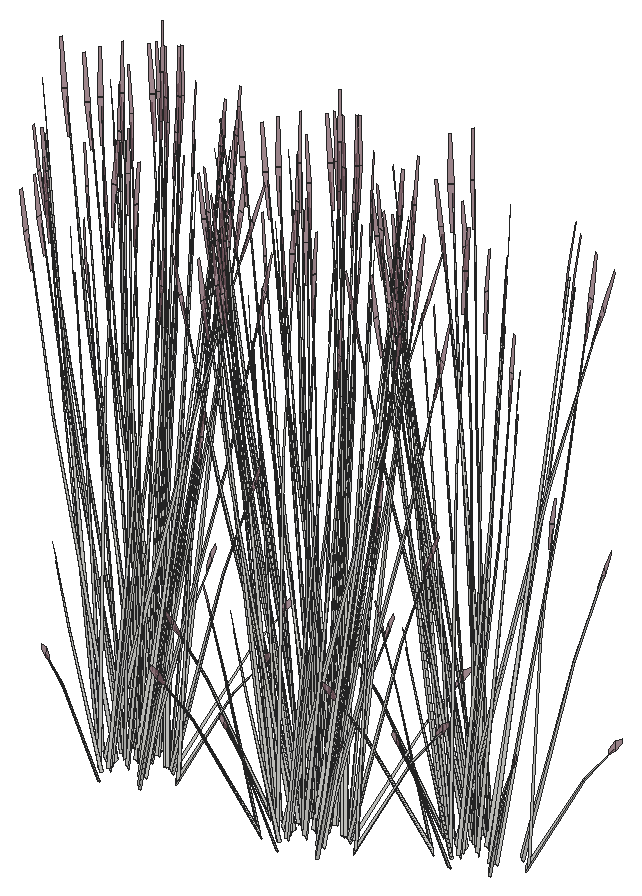
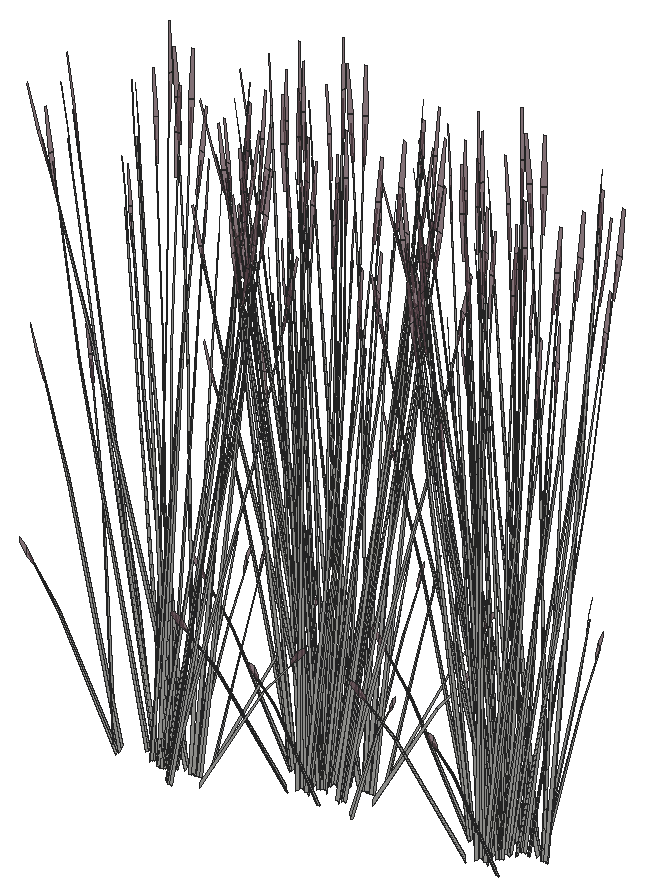
# SketchUp Ruby script. Lengths in inches.
U = 1.inch
M = Sketchup.active_model
def pt(a) = Geom::Point3d.new(a.map { |v| v * U })
def face(e, loops, mat)
  f = e.add_face(loops[0].map { |a| pt(a) })
  loops[1..].each { |l| e.add_face(l.map { |a| pt(a) }).erase! }
  f.material = f.back_material = mat if mat
  f
end
# faces: each face lists its corners as indices into pts; further lists are holes
def faces(e, pts, list, mat = nil) = list.each { |f| face(e, (f[0].is_a?(Array) ? f : [f]).map { |l| l.map { |i| pts[i] } }, mat) }
# xy, xz, yz: faces in a plane at the given z, y or x. An outline is a flat list of corners, or four numbers for a rectangle; further outlines are holes
def ring(l) = l.size == 4 ? [[l[0], l[1]], [l[2], l[1]], [l[2], l[3]], [l[0], l[3]]] : l.each_slice(2).to_a
def flat(e, list, mat, &to3) = list.each { |f| face(e, (f[0].is_a?(Array) ? f : [f]).map { |l| ring(l).map { |u, v| to3.(u, v) } }, mat) }
def xy(e, z, list, mat = nil) = flat(e, list, mat) { |x, y| [x, y, z] }
def xz(e, y, list, mat = nil) = flat(e, list, mat) { |x, z| [x, y, z] }
def yz(e, x, list, mat = nil) = flat(e, list, mat) { |y, z| [x, y, z] }
def lines(e, pts, list) = list.each { |a, b| e.add_line(pt(pts[a]), pt(pts[b])) }
# prism: a flat outline (further loops are holes) pulled along v
def prism(e, loops, v, mat = nil)
  f = face(e, loops, mat); d = Geom::Vector3d.new(v.map { |x| x * U })
  f.pushpull(f.normal.samedirection?(d) ? d.length : -d.length)
end
def box(e, o, s, mat = nil) = prism(e, [[o, [o[0] + s[0], o[1], o[2]], [o[0] + s[0], o[1] + s[1], o[2]], [o[0], o[1] + s[1], o[2]]]], [0, 0, s[2]], mat)
def at(x, y, z, deg = 0) = Geom::Transformation.translation(pt([x, y, z])) * Geom::Transformation.rotation(ORIGIN, Z_AXIS, deg.degrees)
def axes(o, x, y, z) = Geom::Transformation.new([*x, 0, *y, 0, *z, 0, *pt(o).to_a, 1])
def part(name) = M.definitions.add(name)
# library, detail: a bought-in or finely detailed component or shape, given as its bounding box
def library(name, o, s) = part(name).tap { |d| box(d.entities, o, s) }
def detail(e, o, s) = box(e.add_group.entities, o, s)
def put(e, d, t, mat = nil) = e.add_instance(d, t).tap { |i| i.material = mat if mat }
def group(e, t, mat = nil) = e.add_group.tap { |g| g.transformation = t; g.material = mat if mat }.entities
root = M.entities
M.materials.add("LightPink_Translucent").color = [144, 107, 117]
M.materials["LightPink_Translucent"].alpha = 0.75
c1 = part("blade")
p = [[2.15,0.21,22],[0,0.17,0],[0.09,0.45,0],[2.18,0.31,22],[2.29,0.31,22],[0.38,0.45,0],
  [2.48,0.24,33],[2.49,0.24,33],[2.48,0.22,33]]
faces(c1.entities,p,[[0,1,2,3],[4,5,2,3],[6,3,4,7],[8,0,3,6]])
c2 = part("seeds")
p = [[0.3,-0.1,1.38],[-0.01,-0.03,1.59],[-0.01,-0.03,0.03],[0.14,-0.07,-0.07],[0.29,-0.03,3],[0.15,0.01,3.11]]
faces(c2.entities,p,[[0,1,2,3],[1,0,4,5]],"LightPink_Translucent")
c3 = part("blade with seeds")
put(c3.entities,c1,at(0,0,0))
put(c3.entities,c2,axes([2.4,0.25,30.99],[1.5799,-0.05474,1.17369],[-0.12525,1.92788,0.29478],[-0.07173,-0.02425,1.56792]))
put(root,c3,axes([362.03,53.35,257.33],[-0.70674,0.51372,0.30756],[-0.70717,-0.50832,-0.36492],[-0.02468,-0.14589,1.64885]))
put(root,c3,axes([365.23,54.6,257.46],[-0.74193,-0.49181,-0.25192],[0.6243,-0.55226,0.5513],[-0.19979,0.05753,1.68216]))
put(root,c3,axes([363.88,54.13,257.21],[-0.45644,-0.51287,-0.44739],[0.69137,-0.36116,0.21531],[-0.14771,-0.06346,1.43643]))
put(root,c3,axes([364.85,54.5,257.21],[-0.82508,0.03772,-0.44739],[-0.07462,-0.62614,0.21531],[-0.14771,0.06346,1.43643]))
put(root,c3,axes([363.94,54.42,257.4375],[0.20138,-0.72405,-0.23429],[0.95485,0.12621,0.51271],[-0.16685,-0.09999,1.5644]))
put(root,c3,axes([365.72,56.11,257.02],[-0.7111,0.30552,-0.49651],[-0.42504,-0.54784,0],[-0.16196,0.06958,1.57504]))
put(root,c3,axes([361.51,53.07,257.02],[0,-0.61104,-0.49651],[0.85008,0,0],[0,-0.13917,1.57504]))
put(root,c3,axes([365.76,55.95,257.19],[-0.46912,-0.61443,-0.05142],[0.79476,-0.34146,0.51607],[-0.19584,0.0585,1.6363]))
put(root,c3,axes([365.55,55.87,257.03],[-0.70886,-0.15119,-0.30978],[0.17848,-0.53243,0.30978],[-0.1429,0.0614,1.38974]))
put(root,c3,axes([363.73,53.77,257.67],[-0.85568,-0.29155,-0.29095],[0.41201,-0.61537,-0.50002],[-0.02689,-0.15109,1.59708]))
put(root,c3,axes([365.43,54.33,257.67],[0.08854,0.69723,-0.29095],[-0.92215,0.04216,-0.50002],[-0.16238,0.09287,1.59708]))
put(root,c3,axes([363.35,53.15,257.1],[-0.31203,-0.62659,-0.69835],[0.89884,-0.22566,-0.18329],[-0.03449,-0.21218,1.54149]))
put(root,c3,axes([361.87,53.08,257.03],[0.53038,-0.38124,-0.30978],[0.53038,0.38124,0.30978],[0,-0.1228,1.38974]))
put(root,c3,axes([364.27,50.62,257.13],[-0.52505,0.35054,-0.03893],[-0.48109,-0.38392,-0.17649],[-0.03387,-0.10878,0.58215]))
put(root,c3,axes([364.59,55.33,257.2],[-0.76598,-0.27433,0],[0.36864,-0.57001,0],[0,0,1.62707]))
put(root,c3,axes([366.36,56.02,257.375],[0.47504,0.61229,0],[-0.79476,0.34146,-0.51607],[-0.18101,0.07777,1.63711]))
put(root,c3,axes([365.4,54.01,257.3],[-0.70674,-0.52593,-0.06131],[0.70717,-0.52625,0],[-0.02468,-0.01837,1.75571]))
put(root,c3,axes([365.78,55.63,257.33],[0.95122,0.19861,0.30756],[-0.23797,0.7099,-0.36492],[-0.15744,0.08885,1.64885]))
put(root,c3,axes([364.4,50.1875,256.49],[-0.12744,0.02202,1.76342],[-0.70477,-0.24781,-0.26939],[0.01183,-0.2067,0.30037]))
put(root,c3,axes([363.82,53.32,257.21],[0.36864,-0.55059,-0.44739],[0.76598,0.26498,0.21531],[0,-0.12692,1.43643]))
put(root,c3,axes([364.76,55.09,257.2],[-0.24791,-0.5268,0],[0.70791,-0.18448,0],[0,0,1.54371]))
put(root,c3,axes([363.86,56.2,256.49],[0.12297,-0.03325,1.76342],[0.73967,0.18301,-0.26939],[0.02163,0.20626,0.30037]))
put(root,c3,axes([365.76,54.05,257.21],[-0.36864,0.55059,-0.44739],[-0.76598,-0.26498,0.21531],[0,0.12692,1.43643]))
put(root,c3,axes([365.16,53.46,257.21],[0,-0.70701,0],[0.95008,0,0],[0,0,1.79456]))
put(root,c3,axes([365.64,53.74,257.29],[0,0.70667,-0.05637],[-0.95008,0,0],[0,0.02221,1.79368]))
put(root,c3,axes([365.18,55.11,257.29],[0.33034,0.70197,-0.06012],[-0.94388,0.24598,0],[0.01154,0.02451,1.72173]))
put(root,c3,axes([363.22,51.35,257.375],[-0.47504,-0.61229,0],[0.79476,-0.34146,-0.51607],[0.18101,-0.07777,1.63711]))
put(root,c3,axes([367.91,54.19,257.2],[-0.94962,-0.00489,-0.04976],[0,-0.68292,0.49943],[-0.02984,0.15546,1.58352]))
put(root,c3,axes([365.79,53.89,257.21],[0.53038,0.39469,0],[-0.53038,0.39469,0],[0,0,1.69266]))
put(root,c3,axes([365.46,55.34,257.2],[0.76598,0.27433,0],[-0.36864,0.57001,0],[0,0,1.74954]))
put(root,c3,axes([367.71,54.29,257.03],[-0.53038,0.38124,-0.30978],[-0.53038,-0.38124,0.30978],[0,0.1228,1.38974]))
put(root,c3,axes([366.2,54.22,257.09],[0.2786,0.55945,-0.69212],[-0.80253,0.20149,-0.18165],[0.03079,0.18945,1.52773]))
put(root,c3,axes([365.8,53.62,257.21],[0.85008,0,0],[0,0.63259,0],[0,0,1.78407]))
put(root,c3,axes([364.16,53.04,257.67],[-0.08854,-0.69723,-0.29095],[0.92215,-0.04216,-0.50002],[0.16238,-0.09287,1.59708]))
put(root,c3,axes([365.86,53.6,257.67],[0.85568,0.29155,-0.29095],[-0.41201,0.61537,-0.50002],[0.02689,0.15109,1.59708]))
put(root,c3,axes([364.03,51.5,257.03],[0.70886,0.15119,-0.30978],[-0.17848,0.53243,0.30978],[0.1429,-0.0614,1.38974]))
put(root,c3,axes([368.08,54.3,257.02],[0,0.61104,-0.49651],[-0.85008,0,0],[0,0.13917,1.57504]))
put(root,c3,axes([363.87,51.26,257.02],[0.7111,-0.30552,-0.49651],[0.42504,0.54784,0],[0.16196,-0.06958,1.57504]))
put(root,c3,axes([365.69,55.02,257.18],[0.79769,-0.20732,-0.19198],[0.2803,0.59721,0.00008],[0.08805,-0.02292,1.73897]))
put(root,c3,axes([365.71,53.24,257.21],[0.45644,0.51287,-0.44739],[-0.69137,0.36116,0.21531],[0.14771,0.06346,1.43643]))
put(root,c3,axes([364.71,52.51,257.06],[0.51177,-0.45928,-0.62353],[0.63575,0.41646,-0.16365],[0.20507,-0.11457,1.37633]))
put(root,c3,axes([366.96,52.1,257.03],[0.17848,0.53243,-0.30978],[-0.70886,0.15119,0.30978],[0.1429,0.0614,1.38974]))
put(root,c3,axes([368.29,53.84,257.375],[0.95008,0,0],[0,0.68292,-0.51607],[0,0.15554,1.63711]))
put(root,c3,axes([365.22,52.95,257.67],[0.76714,-0.40567,-0.29095],[0.51013,0.57321,-0.50002],[0.18927,0.05821,1.59708]))
put(root,c3,axes([363.28,52.59,256.59],[-0.74787,0.24464,1.28929],[-0.23804,-0.70192,0.50096],[0.45924,0.01168,1.46642]))
put(root,c3,axes([366.72,51.51,257.375],[0.47504,-0.61229,0],[0.79476,0.34146,-0.51607],[0.18101,0.07777,1.63711]))
put(root,c3,axes([367.52,51.24,256.49],[-0.11372,-0.04814,1.76342],[-0.29211,-0.53779,-0.26939],[0.19706,-0.14594,0.30037]))
put(root,c3,axes([367.15,51.875,257.02],[0.7111,0.30552,-0.49651],[-0.42504,0.54784,0],[0.16196,0.06958,1.57504]))
put(root,c3,axes([367.12,56.22,256.49],[0.05536,-0.08822,1.76342],[0.69692,-0.25981,-0.26939],[0.21129,0.13447,0.30037]))
put(root,c3,axes([366.12,53.05,257.06],[0.79037,0.10018,-0.62353],[-0.16679,0.61794,-0.16365],[0.23587,0.07488,1.37633]))
put(root,c3,axes([369.48,53.41,257.26],[-0.47106,-0.39072,-0.06488],[0.51591,-0.35801,-0.29416],[0.14618,-0.02521,0.97024]))
put(root,c3,axes([378.5625,53.45,256.49],[0.01927,0.0963,1.76342],[-0.38846,0.5029,-0.26939],[-0.27592,-0.02535,0.30037]))
put(root,c3,axes([368.59,53.93,256.98],[-0.48937,0.07333,1.41583],[-0.07789,-0.58369,0.08104],[0.34275,-0.08835,0.80566]))
put(root,c3,axes([369.125,53.55,256.49],[-0.03971,-0.09277,1.76342],[0.27541,-0.54264,-0.26939],[0.27782,-0.00781,0.30037]))
put(root,c3,axes([378.35,56.15,256.49],[0.10192,0.06105,1.76342],[0.17281,0.56562,-0.26939],[-0.22588,0.12062,0.30037]))
put(root,c3,axes([381.1,54.32,257.06],[-0.79037,-0.10018,-0.62353],[0.16679,-0.61794,-0.16365],[-0.23587,-0.07488,1.37633]))
put(root,c3,axes([380.07,55.49,257.02],[-0.7111,-0.30552,-0.49651],[0.42504,-0.54784,0],[-0.16196,-0.06958,1.57504]))
put(root,c3,axes([379.75,50.94,256.49],[-0.0736,0.08049,1.76342],[-0.74378,0.17355,-0.26939],[-0.17968,-0.15788,0.30037]))
put(root,c3,axes([380.5,55.86,257.375],[-0.47504,0.61229,0],[-0.79476,-0.34146,-0.51607],[-0.18101,-0.07777,1.63711]))
put(root,c3,axes([379.29,51.25,257.13],[-0.21918,0.49894,-0.03893],[-0.6746,-0.15348,-0.17649],[-0.10242,-0.08161,0.58215]))
put(root,c3,axes([382,54.42,257.67],[-0.76714,0.40567,-0.29095],[-0.51013,-0.57321,-0.50002],[-0.18927,-0.05821,1.59708]))
put(root,c3,axes([378.93,53.53,257.375],[-0.95008,0,0],[0,-0.68292,-0.51607],[0,-0.15554,1.63711]))
put(root,c3,axes([380.26,55.27,257.03],[-0.17848,-0.53243,-0.30978],[0.70886,-0.15119,0.30978],[-0.1429,-0.0614,1.38974]))
put(root,c3,axes([382.51,54.86,257.06],[-0.51177,0.45928,-0.62353],[-0.63575,-0.41646,-0.16365],[-0.20507,0.11457,1.37633]))
put(root,c3,axes([379.67,53.35,257.33],[-0.70674,0.51372,0.30756],[-0.70717,-0.50832,-0.36492],[-0.02468,-0.14589,1.64885]))
put(root,c3,axes([382.86,54.6,257.46],[-0.74193,-0.49181,-0.25192],[0.6243,-0.55226,0.5513],[-0.19979,0.05753,1.68216]))
put(root,c3,axes([381.51,54.13,257.21],[-0.45644,-0.51287,-0.44739],[0.69137,-0.36116,0.21531],[-0.14771,-0.06346,1.43643]))
put(root,c3,axes([382.49,54.5,257.21],[-0.82508,0.03772,-0.44739],[-0.07462,-0.62614,0.21531],[-0.14771,0.06346,1.43643]))
put(root,c3,axes([381.58,54.42,257.4375],[0.20138,-0.72405,-0.23429],[0.95485,0.12621,0.51271],[-0.16685,-0.09999,1.5644]))
put(root,c3,axes([383.35,56.11,257.02],[-0.7111,0.30552,-0.49651],[-0.42504,-0.54784,0],[-0.16196,0.06958,1.57504]))
put(root,c3,axes([379.14,53.07,257.02],[0,-0.61104,-0.49651],[0.85008,0,0],[0,-0.13917,1.57504]))
put(root,c3,axes([383.4,55.95,257.19],[-0.46912,-0.61443,-0.05142],[0.79476,-0.34146,0.51607],[-0.19584,0.0585,1.6363]))
put(root,c3,axes([383.19,55.87,257.03],[-0.70886,-0.15119,-0.30978],[0.17848,-0.53243,0.30978],[-0.1429,0.0614,1.38974]))
put(root,c3,axes([381.36,53.77,257.67],[-0.85568,-0.29155,-0.29095],[0.41201,-0.61537,-0.50002],[-0.02689,-0.15109,1.59708]))
put(root,c3,axes([383.0625,54.33,257.67],[0.08854,0.69723,-0.29095],[-0.92215,0.04216,-0.50002],[-0.16238,0.09287,1.59708]))
put(root,c3,axes([380.98,53.15,257.1],[-0.31203,-0.62659,-0.69835],[0.89884,-0.22566,-0.18329],[-0.03449,-0.21218,1.54149]))
put(root,c3,axes([379.51,53.08,257.03],[0.53038,-0.38124,-0.30978],[0.53038,0.38124,0.30978],[0,-0.1228,1.38974]))
put(root,c3,axes([381.9,50.62,257.13],[-0.52505,0.35054,-0.03893],[-0.48109,-0.38392,-0.17649],[-0.03387,-0.10878,0.58215]))
put(root,c3,axes([382.22,55.33,257.2],[-0.76598,-0.27433,0],[0.36864,-0.57001,0],[0,0,1.62707]))
put(root,c3,axes([384,56.02,257.375],[0.47504,0.61229,0],[-0.79476,0.34146,-0.51607],[-0.18101,0.07777,1.63711]))
put(root,c3,axes([383.03,54.01,257.3],[-0.70674,-0.52593,-0.06131],[0.70717,-0.52625,0],[-0.02468,-0.01837,1.75571]))
put(root,c3,axes([383.42,55.63,257.33],[0.95122,0.19861,0.30756],[-0.23797,0.7099,-0.36492],[-0.15744,0.08885,1.64885]))
put(root,c3,axes([382.03,50.1875,256.49],[-0.12744,0.02202,1.76342],[-0.70477,-0.24781,-0.26939],[0.01183,-0.2067,0.30037]))
put(root,c3,axes([381.46,53.32,257.21],[0.36864,-0.55059,-0.44739],[0.76598,0.26498,0.21531],[0,-0.12692,1.43643]))
put(root,c3,axes([382.4,55.09,257.2],[-0.24791,-0.5268,0],[0.70791,-0.18448,0],[0,0,1.54371]))
put(root,c3,axes([381.5,56.2,256.49],[0.12297,-0.03325,1.76342],[0.73967,0.18301,-0.26939],[0.02163,0.20626,0.30037]))
put(root,c3,axes([383.4,54.05,257.21],[-0.36864,0.55059,-0.44739],[-0.76598,-0.26498,0.21531],[0,0.12692,1.43643]))
put(root,c3,axes([382.8,53.46,257.21],[0,-0.70701,0],[0.95008,0,0],[0,0,1.79456]))
put(root,c3,axes([383.27,53.74,257.29],[0,0.70667,-0.05637],[-0.95008,0,0],[0,0.02221,1.79368]))
put(root,c3,axes([382.82,55.11,257.29],[0.33034,0.70197,-0.06012],[-0.94388,0.24598,0],[0.01154,0.02451,1.72173]))
put(root,c3,axes([380.86,51.35,257.375],[-0.47504,-0.61229,0],[0.79476,-0.34146,-0.51607],[0.18101,-0.07777,1.63711]))
put(root,c3,axes([385.55,54.19,257.2],[-0.94962,-0.00489,-0.04976],[0,-0.68292,0.49943],[-0.02984,0.15546,1.58352]))
put(root,c3,axes([383.42,53.89,257.21],[0.53038,0.39469,0],[-0.53038,0.39469,0],[0,0,1.69266]))
put(root,c3,axes([383.09,55.34,257.2],[0.76598,0.27433,0],[-0.36864,0.57001,0],[0,0,1.74954]))
put(root,c3,axes([385.35,54.29,257.03],[-0.53038,0.38124,-0.30978],[-0.53038,-0.38124,0.30978],[0,0.1228,1.38974]))
put(root,c3,axes([383.83,54.22,257.09],[0.2786,0.55945,-0.69212],[-0.80253,0.20149,-0.18165],[0.03079,0.18945,1.52773]))
put(root,c3,axes([383.44,53.62,257.21],[0.85008,0,0],[0,0.63259,0],[0,0,1.78407]))
put(root,c3,axes([381.79,53.04,257.67],[-0.08854,-0.69723,-0.29095],[0.92215,-0.04216,-0.50002],[0.16238,-0.09287,1.59708]))
put(root,c3,axes([383.49,53.6,257.67],[0.85568,0.29155,-0.29095],[-0.41201,0.61537,-0.50002],[0.02689,0.15109,1.59708]))
put(root,c3,axes([381.67,51.5,257.03],[0.70886,0.15119,-0.30978],[-0.17848,0.53243,0.30978],[0.1429,-0.0614,1.38974]))
put(root,c3,axes([385.71,54.3,257.02],[0,0.61104,-0.49651],[-0.85008,0,0],[0,0.13917,1.57504]))
put(root,c3,axes([381.5,51.26,257.02],[0.7111,-0.30552,-0.49651],[0.42504,0.54784,0],[0.16196,-0.06958,1.57504]))
put(root,c3,axes([390.69,59.68,256.49],[0.01927,0.0963,1.76342],[-0.38846,0.5029,-0.26939],[-0.27592,-0.02535,0.30037]))
put(root,c3,axes([383.33,55.02,257.18],[0.79769,-0.20732,-0.19198],[0.2803,0.59721,0.00008],[0.08805,-0.02292,1.73897]))
put(root,c3,axes([383.34,53.24,257.21],[0.45644,0.51287,-0.44739],[-0.69137,0.36116,0.21531],[0.14771,0.06346,1.43643]))
put(root,c3,axes([382.35,52.51,257.06],[0.51177,-0.45928,-0.62353],[0.63575,0.41646,-0.16365],[0.20507,-0.11457,1.37633]))
put(root,c3,axes([384.59,52.1,257.03],[0.17848,0.53243,-0.30978],[-0.70886,0.15119,0.30978],[0.1429,0.0614,1.38974]))
put(root,c3,axes([385.93,53.84,257.375],[0.95008,0,0],[0,0.68292,-0.51607],[0,0.15554,1.63711]))
put(root,c3,axes([382.86,52.95,257.67],[0.76714,-0.40567,-0.29095],[0.51013,0.57321,-0.50002],[0.18927,0.05821,1.59708]))
put(root,c3,axes([393.23,60.55,257.06],[-0.79037,-0.10018,-0.62353],[0.16679,-0.61794,-0.16365],[-0.23587,-0.07488,1.37633]))
put(root,c3,axes([380.92,52.59,256.59],[-0.74787,0.24464,1.28929],[-0.23804,-0.70192,0.50096],[0.45924,0.01168,1.46642]))
put(root,c3,axes([392.2,61.72,257.02],[-0.7111,-0.30552,-0.49651],[0.42504,-0.54784,0],[-0.16196,-0.06958,1.57504]))
put(root,c3,axes([391.88,57.17,256.49],[-0.0736,0.08049,1.76342],[-0.74378,0.17355,-0.26939],[-0.17968,-0.15788,0.30037]))
put(root,c3,axes([384.36,51.51,257.375],[0.47504,-0.61229,0],[0.79476,0.34146,-0.51607],[0.18101,0.07777,1.63711]))
put(root,c3,axes([385.15,51.24,256.49],[-0.11372,-0.04814,1.76342],[-0.29211,-0.53779,-0.26939],[0.19706,-0.14594,0.30037]))
put(root,c3,axes([384.79,51.875,257.02],[0.7111,0.30552,-0.49651],[-0.42504,0.54784,0],[0.16196,0.06958,1.57504]))
put(root,c3,axes([384.75,56.22,256.49],[0.05536,-0.08822,1.76342],[0.69692,-0.25981,-0.26939],[0.21129,0.13447,0.30037]))
put(root,c3,axes([391.42,57.48,257.13],[-0.21918,0.49894,-0.03893],[-0.6746,-0.15348,-0.17649],[-0.10242,-0.08161,0.58215]))
put(root,c3,axes([383.75,53.05,257.06],[0.79037,0.10018,-0.62353],[-0.16679,0.61794,-0.16365],[0.23587,0.07488,1.37633]))
put(root,c3,axes([387.12,53.41,257.26],[-0.47106,-0.39072,-0.06488],[0.51591,-0.35801,-0.29416],[0.14618,-0.02521,0.97024]))
put(root,c3,axes([391.06,59.76,257.375],[-0.95008,0,0],[0,-0.68292,-0.51607],[0,-0.15554,1.63711]))
put(root,c3,axes([392.39,61.49,257.03],[-0.17848,-0.53243,-0.30978],[0.70886,-0.15119,0.30978],[-0.1429,-0.0614,1.38974]))
put(root,c3,axes([391.8,59.58,257.33],[-0.70674,0.51372,0.30756],[-0.70717,-0.50832,-0.36492],[-0.02468,-0.14589,1.64885]))
put(root,c3,axes([393.64,60.35,257.21],[-0.45644,-0.51287,-0.44739],[0.69137,-0.36116,0.21531],[-0.14771,-0.06346,1.43643]))
put(root,c3,axes([393.71,60.65,257.4375],[0.20138,-0.72405,-0.23429],[0.95485,0.12621,0.51271],[-0.16685,-0.09999,1.5644]))
put(root,c3,axes([391.27,59.29,257.02],[0,-0.61104,-0.49651],[0.85008,0,0],[0,-0.13917,1.57504]))
put(root,c3,axes([386.23,53.93,256.98],[-0.48937,0.07333,1.41583],[-0.07789,-0.58369,0.08104],[0.34275,-0.08835,0.80566]))
put(root,c3,axes([386.76,53.55,256.49],[-0.03971,-0.09277,1.76342],[0.27541,-0.54264,-0.26939],[0.27782,-0.00781,0.30037]))
put(root,c3,axes([393.49,60,257.67],[-0.85568,-0.29155,-0.29095],[0.41201,-0.61537,-0.50002],[-0.02689,-0.15109,1.59708]))
put(root,c3,axes([393.11,59.38,257.1],[-0.31203,-0.62659,-0.69835],[0.89884,-0.22566,-0.18329],[-0.03449,-0.21218,1.54149]))
put(root,c3,axes([391.64,59.31,257.03],[0.53038,-0.38124,-0.30978],[0.53038,0.38124,0.30978],[0,-0.1228,1.38974]))
put(root,c3,axes([394.03,56.84,257.13],[-0.52505,0.35054,-0.03893],[-0.48109,-0.38392,-0.17649],[-0.03387,-0.10878,0.58215]))
put(root,c3,axes([393.82,60.3,257.36],[0.96033,0.12874,0.45755],[-0.19544,0.7271,0.17955],[-0.14034,-0.07021,1.58856]))
put(root,c3,axes([395.16,60.24,257.3],[-0.70674,-0.52593,-0.06131],[0.70717,-0.52625,0],[-0.02468,-0.01837,1.75571]))
put(root,c3,axes([394.16,56.41,256.49],[-0.12744,0.02202,1.76342],[-0.70477,-0.24781,-0.26939],[0.01183,-0.2067,0.30037]))
put(root,c3,axes([393.74,59.63,257.36],[0.33034,0.68327,0.45755],[-0.94388,0.2376,0.17955],[0.01154,-0.12555,1.58856]))
put(root,c3,axes([393.59,59.54,257.21],[0.36864,-0.55059,-0.44739],[0.76598,0.26498,0.21531],[0,-0.12692,1.43643]))
put(root,c3,axes([394.93,59.6875,257.21],[0,-0.70701,0],[0.95008,0,0],[0,0,1.79456]))
put(root,c3,axes([392.99,57.58,257.375],[-0.47504,-0.61229,0],[0.79476,-0.34146,-0.51607],[0.18101,-0.07777,1.63711]))
put(root,c3,axes([394.48,59.24,257.36],[-0.62999,0.55453,0.45755],[-0.74845,-0.4895,0.17955],[0.15188,-0.05534,1.58856]))
put(root,c3,axes([393.92,59.27,257.67],[-0.08854,-0.69723,-0.29095],[0.92215,-0.04216,-0.50002],[0.16238,-0.09287,1.59708]))
put(root,c3,axes([393.8,57.73,257.03],[0.70886,0.15119,-0.30978],[-0.17848,0.53243,0.30978],[0.1429,-0.0614,1.38974]))
put(root,c3,axes([393.63,57.49,257.02],[0.7111,-0.30552,-0.49651],[0.42504,0.54784,0],[0.16196,-0.06958,1.57504]))
put(root,c3,axes([394.48,58.74,257.06],[0.51177,-0.45928,-0.62353],[0.63575,0.41646,-0.16365],[0.20507,-0.11457,1.37633]))
put(root,c3,axes([394.99,59.18,257.67],[0.76714,-0.40567,-0.29095],[0.51013,0.57321,-0.50002],[0.18927,0.05821,1.59708]))
put(root,c3,axes([393.05,58.82,256.59],[-0.74787,0.24464,1.28929],[-0.23804,-0.70192,0.50096],[0.45924,0.01168,1.46642]))
put(root,c3,axes([396.49,57.73,257.375],[0.47504,-0.61229,0],[0.79476,0.34146,-0.51607],[0.18101,0.07777,1.63711]))
put(root,c3,axes([397.28,57.47,256.49],[-0.11372,-0.04814,1.76342],[-0.29211,-0.53779,-0.26939],[0.19706,-0.14594,0.30037]))
put(root,c3,axes([396.92,58.1,257.02],[0.7111,0.30552,-0.49651],[-0.42504,0.54784,0],[0.16196,0.06958,1.57504]))
put(root,c3,axes([399.25,59.64,257.26],[-0.47106,-0.39072,-0.06488],[0.51591,-0.35801,-0.29416],[0.14618,-0.02521,0.97024]))
put(root,c3,axes([398.36,60.15,256.98],[-0.48937,0.07333,1.41583],[-0.07789,-0.58369,0.08104],[0.34275,-0.08835,0.80566]))
put(root,c3,axes([398.89,59.77,256.49],[-0.03971,-0.09277,1.76342],[0.27541,-0.54264,-0.26939],[0.27782,-0.00781,0.30037]))
